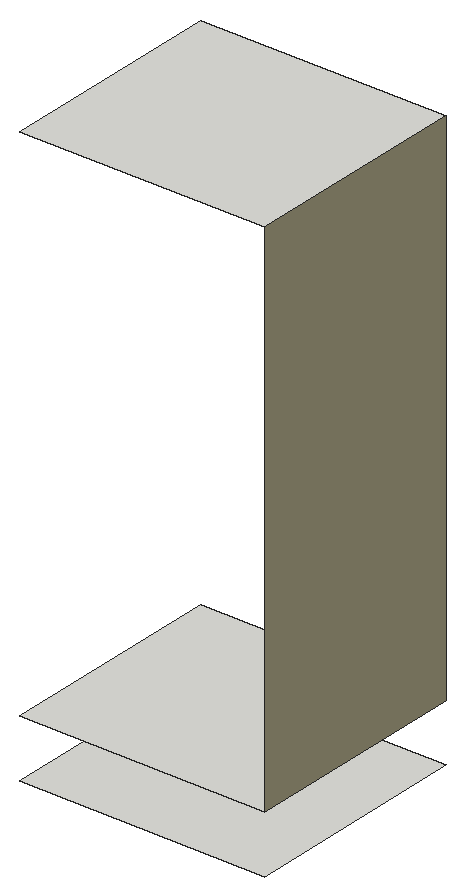
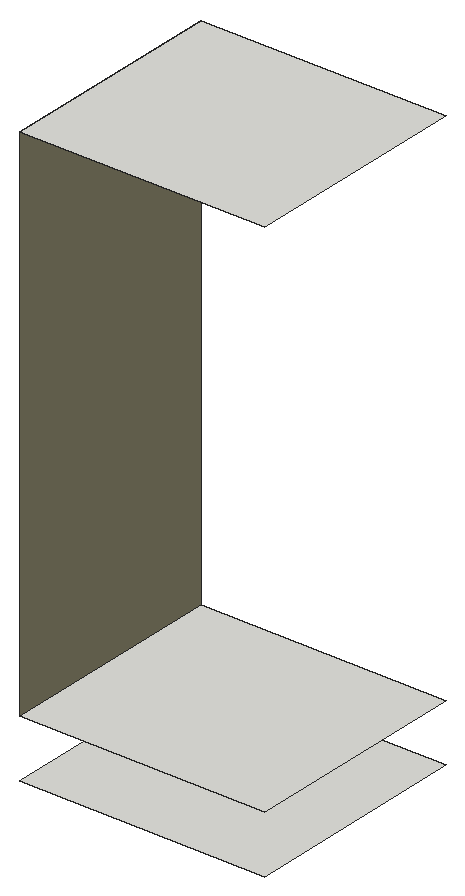
# SketchUp Ruby script. Lengths in inches.
U = 1.inch
M = Sketchup.active_model
def pt(a) = Geom::Point3d.new(a.map { |v| v * U })
def face(e, loops, mat)
  f = e.add_face(loops[0].map { |a| pt(a) })
  loops[1..].each { |l| e.add_face(l.map { |a| pt(a) }).erase! }
  f.material = f.back_material = mat if mat
  f
end
# faces: each face lists its corners as indices into pts; further lists are holes
def faces(e, pts, list, mat = nil) = list.each { |f| face(e, (f[0].is_a?(Array) ? f : [f]).map { |l| l.map { |i| pts[i] } }, mat) }
# xy, xz, yz: faces in a plane at the given z, y or x. An outline is a flat list of corners, or four numbers for a rectangle; further outlines are holes
def ring(l) = l.size == 4 ? [[l[0], l[1]], [l[2], l[1]], [l[2], l[3]], [l[0], l[3]]] : l.each_slice(2).to_a
def flat(e, list, mat, &to3) = list.each { |f| face(e, (f[0].is_a?(Array) ? f : [f]).map { |l| ring(l).map { |u, v| to3.(u, v) } }, mat) }
def xy(e, z, list, mat = nil) = flat(e, list, mat) { |x, y| [x, y, z] }
def xz(e, y, list, mat = nil) = flat(e, list, mat) { |x, z| [x, y, z] }
def yz(e, x, list, mat = nil) = flat(e, list, mat) { |y, z| [x, y, z] }
def lines(e, pts, list) = list.each { |a, b| e.add_line(pt(pts[a]), pt(pts[b])) }
# prism: a flat outline (further loops are holes) pulled along v
def prism(e, loops, v, mat = nil)
  f = face(e, loops, mat); d = Geom::Vector3d.new(v.map { |x| x * U })
  f.pushpull(f.normal.samedirection?(d) ? d.length : -d.length)
end
def box(e, o, s, mat = nil) = prism(e, [[o, [o[0] + s[0], o[1], o[2]], [o[0] + s[0], o[1] + s[1], o[2]], [o[0], o[1] + s[1], o[2]]]], [0, 0, s[2]], mat)
def at(x, y, z, deg = 0) = Geom::Transformation.translation(pt([x, y, z])) * Geom::Transformation.rotation(ORIGIN, Z_AXIS, deg.degrees)
def axes(o, x, y, z) = Geom::Transformation.new([*x, 0, *y, 0, *z, 0, *pt(o).to_a, 1])
def part(name) = M.definitions.add(name)
# library, detail: a bought-in or finely detailed component or shape, given as its bounding box
def library(name, o, s) = part(name).tap { |d| box(d.entities, o, s) }
def detail(e, o, s) = box(e.add_group.entities, o, s)
def put(e, d, t, mat = nil) = e.add_instance(d, t).tap { |i| i.material = mat if mat }
def group(e, t, mat = nil) = e.add_group.tap { |g| g.transformation = t; g.material = mat if mat }.entities
root = M.entities
M.materials.add("[Stone Coursed Rough]").color = [155, 150, 122]
xy(root,92.87,[[281.86,203.17,297.85,217.98]])
xy(root,96.63,[[281.86,203.17,297.85,217.98]])
xy(root,130.875,[[281.86,203.17,297.85,217.98]])
yz(root,297.85,[[203.17,96.63,217.98,130.875]],"[Stone Coursed Rough]")
